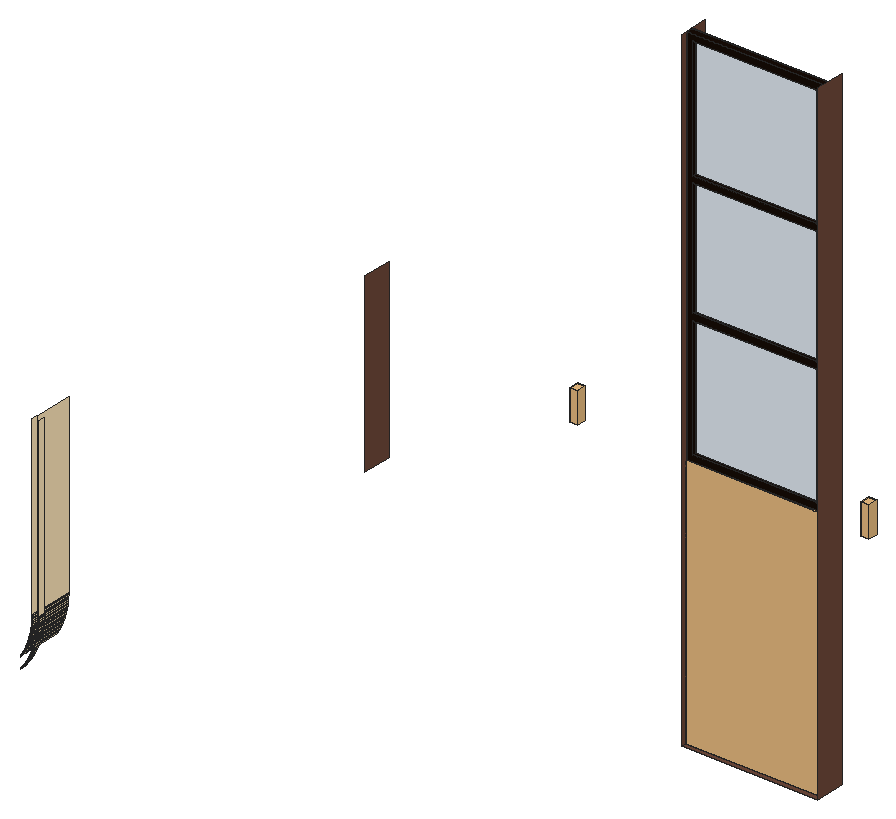
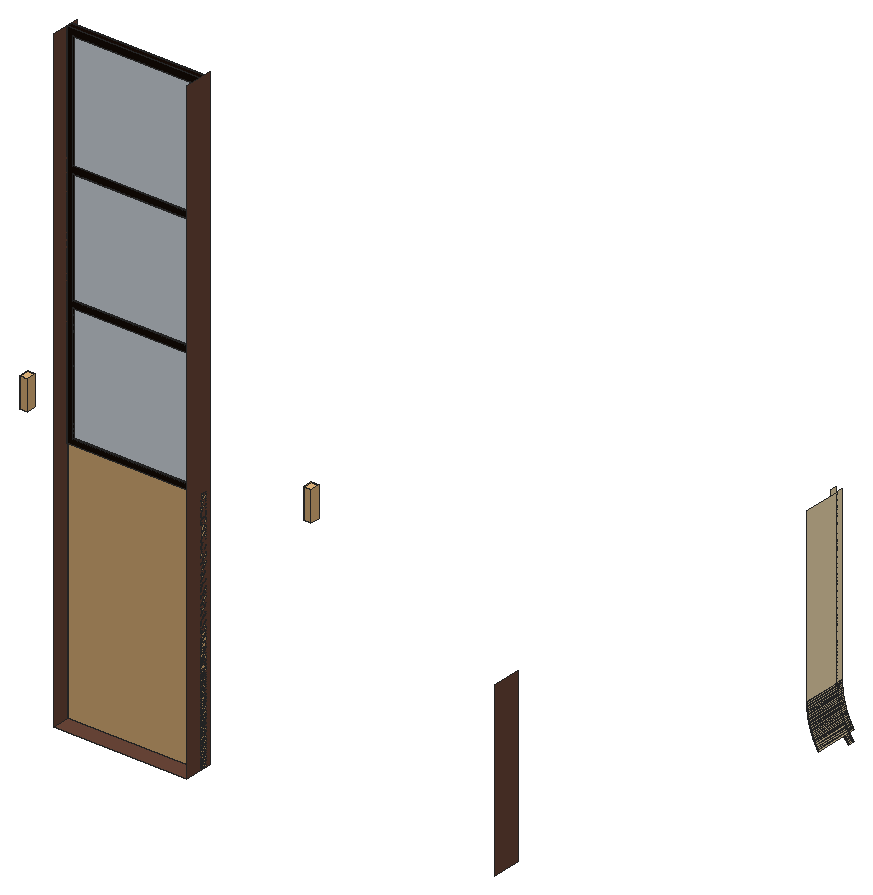
# SketchUp Ruby script. Lengths in inches.
U = 1.inch
M = Sketchup.active_model
def pt(a) = Geom::Point3d.new(a.map { |v| v * U })
def face(e, loops, mat)
  f = e.add_face(loops[0].map { |a| pt(a) })
  loops[1..].each { |l| e.add_face(l.map { |a| pt(a) }).erase! }
  f.material = f.back_material = mat if mat
  f
end
# faces: each face lists its corners as indices into pts; further lists are holes
def faces(e, pts, list, mat = nil) = list.each { |f| face(e, (f[0].is_a?(Array) ? f : [f]).map { |l| l.map { |i| pts[i] } }, mat) }
# xy, xz, yz: faces in a plane at the given z, y or x. An outline is a flat list of corners, or four numbers for a rectangle; further outlines are holes
def ring(l) = l.size == 4 ? [[l[0], l[1]], [l[2], l[1]], [l[2], l[3]], [l[0], l[3]]] : l.each_slice(2).to_a
def flat(e, list, mat, &to3) = list.each { |f| face(e, (f[0].is_a?(Array) ? f : [f]).map { |l| ring(l).map { |u, v| to3.(u, v) } }, mat) }
def xy(e, z, list, mat = nil) = flat(e, list, mat) { |x, y| [x, y, z] }
def xz(e, y, list, mat = nil) = flat(e, list, mat) { |x, z| [x, y, z] }
def yz(e, x, list, mat = nil) = flat(e, list, mat) { |y, z| [x, y, z] }
def lines(e, pts, list) = list.each { |a, b| e.add_line(pt(pts[a]), pt(pts[b])) }
# prism: a flat outline (further loops are holes) pulled along v
def prism(e, loops, v, mat = nil)
  f = face(e, loops, mat); d = Geom::Vector3d.new(v.map { |x| x * U })
  f.pushpull(f.normal.samedirection?(d) ? d.length : -d.length)
end
def box(e, o, s, mat = nil) = prism(e, [[o, [o[0] + s[0], o[1], o[2]], [o[0] + s[0], o[1] + s[1], o[2]], [o[0], o[1] + s[1], o[2]]]], [0, 0, s[2]], mat)
def at(x, y, z, deg = 0) = Geom::Transformation.translation(pt([x, y, z])) * Geom::Transformation.rotation(ORIGIN, Z_AXIS, deg.degrees)
def axes(o, x, y, z) = Geom::Transformation.new([*x, 0, *y, 0, *z, 0, *pt(o).to_a, 1])
def part(name) = M.definitions.add(name)
# library, detail: a bought-in or finely detailed component or shape, given as its bounding box
def library(name, o, s) = part(name).tap { |d| box(d.entities, o, s) }
def detail(e, o, s) = box(e.add_group.entities, o, s)
def put(e, d, t, mat = nil) = e.add_instance(d, t).tap { |i| i.material = mat if mat }
def group(e, t, mat = nil) = e.add_group.tap { |g| g.transformation = t; g.material = mat if mat }.entities
root = M.entities
M.materials.add("1026 AP 7946 SUNNY SIDE UP").color = [254, 231, 186]
M.materials.add("1916 AP K226 Macadamia Cream-N").color = [109, 72, 58]
M.materials.add("[Mirror 02]").color = [228, 237, 245]
M.materials.add("[Wood Veneer 01]").color = [23, 13, 7]
c1 = library("WALL LIGHT 69",[4.19,4.05,-9.3],[4.61,5.7,18.16])
c2 = part("1")
box(c2.entities,[0,-0.47,0],[38,0.47,35.96])
c3 = library("Glass Door",[0,0,0],[72,3.54,96])
xy(root,138,[[305.52,302,347.52,311]],"1916 AP K226 Macadamia Cream-N")
yz(root,177,[[213.1,167.53,215,167.76],[215,167.53,215.1,167.76],[215.1,167.53,227,167.76],[213.1,167.76,215,168],[215,167.76,215.1,168],
  [215.1,167.76,227,168],[213.1,168,215,222],[215,168,215.1,222],[215.1,168,227,222]],"1026 AP 7946 SUNNY SIDE UP")
yz(root,179,[[213.1,167.49,215.1,167.74],[213.1,167.74,215.1,168],[213.1,168,215.1,222]],"1026 AP 7946 SUNNY SIDE UP")
yz(root,189,[[326,162,335,216]],"1916 AP K226 Macadamia Cream-N")
yz(root,305.52,[[302,138,311,333.89]],"1916 AP K226 Macadamia Cream-N")
yz(root,347.52,[[302,138,311,333.89]],"1916 AP K226 Macadamia Cream-N")
p = [[173.42,213.1,151.9],[173.42,215.1,151.9],[173.58,215.1,152.1],[173.58,213.1,152.1],[173.73,215.1,152.31],[173.73,213.1,152.31],
  [173.88,215.1,152.51],[173.88,213.1,152.51],[174.03,215.1,152.72],[174.03,213.1,152.72],[174.18,215.1,152.92],[174.18,213.1,152.92],
  [174.33,215.1,153.13],[174.33,213.1,153.13],[174.48,215.1,153.34],[174.48,213.1,153.34],[174.62,215.1,153.56],[174.62,213.1,153.56],
  [174.76,215.1,153.77],[174.76,213.1,153.77],[174.9,215.1,153.98],[174.9,213.1,153.98],[175.03,215.1,154.2],[175.03,213.1,154.2],
  [175.17,215.1,154.42],[175.17,213.1,154.42],[175.3,215.1,154.63],[175.3,213.1,154.63],[175.43,215.1,154.85],[175.43,213.1,154.85],
  [175.56,215.1,155.07],[175.56,213.1,155.07],[175.68,215.1,155.3],[175.68,213.1,155.3],[173.46,213.1,155.46],[173.46,215,155.46],
  [173.34,215,155.26],[173.34,213.1,155.26],[175.81,215.1,155.52],[175.81,213.1,155.52],[173.34,227,155.26],[173.34,215.1,155.26],
  [173.46,215.1,155.46],[173.46,227,155.46],[173.59,213.1,155.66],[173.59,215,155.66],[175.93,215.1,155.74],[175.93,213.1,155.74],
  [173.59,215.1,155.66],[173.59,227,155.66],[173.71,213.1,155.86],[173.71,215,155.86],[176.05,215.1,155.97],[176.05,213.1,155.97],
  [173.71,215.1,155.86],[173.71,227,155.86],[173.82,213.1,156.07],[173.82,215,156.07],[173.82,215.1,156.07],[173.82,227,156.07],
  [176.17,215.1,156.2],[176.17,213.1,156.2],[173.94,213.1,156.27],[173.94,215,156.27],[173.94,215.1,156.27],[173.94,227,156.27],
  [176.28,215.1,156.42],[176.28,213.1,156.42],[174.05,213.1,156.48],[174.05,215,156.48],[174.05,215.1,156.48],[174.05,227,156.48],
  [176.39,215.1,156.65],[176.39,213.1,156.65],[174.17,213.1,156.6875],[174.17,215,156.6875],[174.17,215.1,156.6875],[174.17,227,156.6875],
  [174.28,213.1,156.89],[174.28,215,156.89],[176.5,215.1,156.88],[176.5,213.1,156.88],[174.28,215.1,156.89],[174.28,227,156.89],
  [174.38,213.1,157.1],[174.38,215,157.1],[176.61,215.1,157.11],[176.61,213.1,157.11],[174.38,215.1,157.1],[174.38,227,157.1],
  [174.49,213.1,157.31],[174.49,215,157.31],[176.72,215.1,157.35],[176.72,213.1,157.35],[174.49,215.1,157.31],[174.49,227,157.31],
  [174.59,213.1,157.53],[174.59,215,157.53],[176.82,215.1,157.58],[176.82,213.1,157.58],[174.59,215.1,157.53],[174.59,227,157.53],
  [174.7,213.1,157.74],[174.7,215,157.74],[174.7,215.1,157.74],[174.7,227,157.74],[176.92,215.1,157.81],[176.92,213.1,157.81],
  [174.8,213.1,157.95],[174.8,215,157.95],[174.8,215.1,157.95],[174.8,227,157.95],[177.02,215.1,158.05],[177.02,213.1,158.05],
  [174.89,213.1,158.17],[174.89,215,158.17],[174.89,215.1,158.17],[174.89,227,158.17],[177.12,215.1,158.29],[177.12,213.1,158.29],
  [174.99,213.1,158.38],[174.99,215,158.38],[174.99,215.1,158.38],[174.99,227,158.38],[177.21,215.1,158.52],[177.21,213.1,158.52],
  [175.08,213.1,158.6],[175.08,215,158.6],[175.08,215.1,158.6],[175.08,227,158.6],[177.3,215.1,158.76],[177.3,213.1,158.76],
  [175.17,213.1,158.82],[175.17,215,158.82],[175.17,215.1,158.82],[175.17,227,158.82],[175.26,213.1,159.03],[175.26,215,159.03],
  [177.39,215.1,159],[177.39,213.1,159],[175.26,215.1,159.03],[175.26,227,159.03],[175.35,213.1,159.25],[175.35,215,159.25],
  [177.48,215.1,159.24],[177.48,213.1,159.24],[175.35,215.1,159.25],[175.35,227,159.25],[177.56,215.1,159.48],[177.56,213.1,159.48],
  [175.43,213.1,159.47],[175.43,215,159.47],[175.43,215.1,159.47],[175.43,227,159.47],[175.52,213.1,159.69],[175.52,215,159.69],
  [177.65,215.1,159.72],[177.65,213.1,159.72],[175.52,215.1,159.69],[175.52,227,159.69],[175.6,213.1,159.91],[175.6,215,159.91],
  [177.73,215.1,159.97],[177.73,213.1,159.97],[175.6,215.1,159.91],[175.6,227,159.91],[175.68,213.1,160.14],[175.68,215,160.14],
  [175.68,215.1,160.14],[175.68,227,160.14],[177.81,215.1,160.21],[177.81,213.1,160.21],[175.75,213.1,160.36],[175.75,215,160.36],
  [175.75,215.1,160.36],[175.75,227,160.36],[177.88,215.1,160.45],[177.88,213.1,160.45],[175.83,213.1,160.58],[175.83,215,160.58],
  [175.83,215.1,160.58],[175.83,227,160.58],[177.95,215.1,160.7],[177.95,213.1,160.7],[175.9,213.1,160.81],[175.9,215,160.81],
  [175.9,215.1,160.81],[175.9,227,160.81],[178.02,215.1,160.94],[178.02,213.1,160.94],[175.97,213.1,161.03],[175.97,215,161.03],
  [175.97,215.1,161.03],[175.97,227,161.03],[178.09,215.1,161.1875],[178.09,213.1,161.1875],[176.03,213.1,161.26],[176.03,215,161.26],
  [176.03,215.1,161.26],[176.03,227,161.26],[178.16,215.1,161.44],[178.16,213.1,161.44],[176.1,213.1,161.49],[176.1,215,161.49],
  [176.1,215.1,161.49],[176.1,227,161.49],[178.22,215.1,161.68],[178.22,213.1,161.68],[176.16,213.1,161.71],[176.16,215,161.71],
  [176.16,215.1,161.71],[176.16,227,161.71],[176.22,213.1,161.94],[176.22,215,161.94],[178.28,215.1,161.93],[178.28,213.1,161.93],
  [176.22,215.1,161.94],[176.22,227,161.94],[176.28,213.1,162.17],[176.28,215,162.17],[178.34,215.1,162.18],[178.34,213.1,162.18],
  [176.28,215.1,162.17],[176.28,227,162.17],[176.34,213.1,162.4],[176.34,215,162.4],[178.4,215.1,162.43],[178.4,213.1,162.43],
  [176.34,215.1,162.4],[176.34,227,162.4],[176.39,213.1,162.625],[176.39,215,162.625],[178.45,215.1,162.68],[178.45,213.1,162.68],
  [176.39,215.1,162.625],[176.39,227,162.625],[176.44,213.1,162.86],[176.44,215,162.86],[176.44,215.1,162.86],[176.44,227,162.86],
  [178.5,215.1,162.93],[178.5,213.1,162.93],[176.49,213.1,163.09],[176.49,215,163.09],[178.55,215.1,163.18],[178.55,213.1,163.18],
  [176.49,215.1,163.09],[176.49,227,163.09],[176.54,213.1,163.32],[176.54,215,163.32],[176.54,215.1,163.32],[176.54,227,163.32],
  [178.6,215.1,163.43],[178.6,213.1,163.43],[176.58,213.1,163.55],[176.58,215,163.55],[176.58,215.1,163.55],[176.58,227,163.55],
  [178.64,215.1,163.68],[178.64,213.1,163.68],[176.625,213.1,163.78],[176.625,215,163.78],[176.625,215.1,163.78],[176.625,227,163.78],
  [178.68,215.1,163.93],[178.68,213.1,163.93],[176.67,213.1,164.01],[176.67,215,164.01],[176.67,215.1,164.01],[176.67,227,164.01],
  [178.72,215.1,164.19],[178.72,213.1,164.19],[176.7,213.1,164.25],[176.7,215,164.25],[176.7,215.1,164.25],[176.7,227,164.25],
  [176.74,213.1,164.48],[176.74,215,164.48],[178.75,215.1,164.4375],[178.75,213.1,164.4375],[176.74,215.1,164.48],[176.74,227,164.48],
  [178.79,215.1,164.69],[178.79,213.1,164.69],[176.77,213.1,164.71],[176.77,215,164.71],[176.77,215.1,164.71],[176.77,227,164.71],
  [176.8,213.1,164.95],[176.8,215,164.95],[178.82,215.1,164.94],[178.82,213.1,164.94],[176.8,215.1,164.95],[176.8,227,164.95],
  [176.83,213.1,165.18],[176.83,215,165.18],[178.85,215.1,165.2],[178.85,213.1,165.2],[176.83,215.1,165.18],[176.83,227,165.18],
  [176.86,213.1,165.41],[176.86,215,165.41],[178.875,215.1,165.45],[178.875,213.1,165.45],[176.86,215.1,165.41],[176.86,227,165.41],
  [176.88,213.1,165.65],[176.88,215,165.65],[176.88,215.1,165.65],[176.88,227,165.65],[178.9,215.1,165.71],[178.9,213.1,165.71],
  [176.91,213.1,165.88],[176.91,215,165.88],[176.91,215.1,165.88],[176.91,227,165.88],[178.92,215.1,165.96],[178.92,213.1,165.96],
  [176.93,213.1,166.12],[176.93,215,166.12],[176.93,215.1,166.12],[176.93,227,166.12],[178.9375,215.1,166.21],[178.9375,213.1,166.21],
  [176.94,213.1,166.35],[176.94,215,166.35],[176.94,215.1,166.35],[176.94,227,166.35],[178.95,215.1,166.47],[178.95,213.1,166.47],
  [176.96,213.1,166.59],[176.96,215,166.59],[176.96,215.1,166.59],[176.96,227,166.59],[178.97,215.1,166.72],[178.97,213.1,166.72],
  [176.97,213.1,166.82],[176.97,215,166.82],[176.97,215.1,166.82],[176.97,227,166.82],[178.98,215.1,166.98],[178.98,213.1,166.98],
  [176.98,213.1,167.06],[176.98,215,167.06],[176.98,215.1,167.06],[176.98,227,167.06],[178.99,215.1,167.23],[178.99,213.1,167.23],
  [176.99,213.1,167.29],[176.99,215,167.29],[176.99,215.1,167.29],[176.99,227,167.29],[179,215.1,167.49],[179,213.1,167.49],
  [177,213.1,167.53],[177,215,167.53],[177,215.1,167.53],[177,227,167.53]]
faces(root,p,[[0,1,2,3],[3,2,4,5],[5,4,6,7],[7,6,8,9],[9,8,10,11],[11,10,12,13],[13,12,14,15],[15,14,16,17],
  [17,16,18,19],[19,18,20,21],[21,20,22,23],[23,22,24,25],[25,24,26,27],[27,26,28,29],[29,28,30,31],[31,30,32,33],
  [34,35,36,37],[33,32,38,39],[40,41,42,43],[44,45,35,34],[39,38,46,47],[42,35,45,48],[43,42,48,49],[50,51,45,44],
  [47,46,52,53],[48,45,51,54],[49,48,54,55],[56,57,51,50],[54,51,57,58],[55,54,58,59],[53,52,60,61],[62,63,57,56],
  [58,57,63,64],[59,58,64,65],[61,60,66,67],[68,69,63,62],[64,63,69,70],[65,64,70,71],[67,66,72,73],[74,75,69,68],
  [70,69,75,76],[71,70,76,77],[78,79,75,74],[73,72,80,81],[76,75,79,82],[77,76,82,83],[84,85,79,78],[81,80,86,87],
  [82,79,85,88],[83,82,88,89],[90,91,85,84],[87,86,92,93],[88,85,91,94],[89,88,94,95],[96,97,91,90],[93,92,98,99],
  [94,91,97,100],[95,94,100,101],[102,103,97,96],[100,97,103,104],[101,100,104,105],[99,98,106,107],[108,109,103,102],[104,103,109,110],
  [105,104,110,111],[107,106,112,113],[114,115,109,108],[110,109,115,116],[111,110,116,117],[113,112,118,119],[120,121,115,114],[116,115,121,122],
  [117,116,122,123],[119,118,124,125],[126,127,121,120],[122,121,127,128],[123,122,128,129],[125,124,130,131],[132,133,127,126],[128,127,133,134],
  [129,128,134,135],[136,137,133,132],[131,130,138,139],[134,133,137,140],[135,134,140,141],[142,143,137,136],[139,138,144,145],[140,137,143,146],
  [141,140,146,147],[145,144,148,149],[150,151,143,142],[146,143,151,152],[147,146,152,153],[154,155,151,150],[149,148,156,157],[152,151,155,158],
  [153,152,158,159],[160,161,155,154],[157,156,162,163],[158,155,161,164],[159,158,164,165],[166,167,161,160],[164,161,167,168],[165,164,168,169],
  [163,162,170,171],[172,173,167,166],[168,167,173,174],[169,168,174,175],[171,170,176,177],[178,179,173,172],[174,173,179,180],[175,174,180,181],
  [177,176,182,183],[184,185,179,178],[180,179,185,186],[181,180,186,187],[183,182,188,189],[190,191,185,184],[186,185,191,192],[187,186,192,193],
  [189,188,194,195],[196,197,191,190],[192,191,197,198],[193,192,198,199],[195,194,200,201],[202,203,197,196],[198,197,203,204],[199,198,204,205],
  [201,200,206,207],[208,209,203,202],[204,203,209,210],[205,204,210,211],[212,213,209,208],[207,206,214,215],[210,209,213,216],[211,210,216,217],
  [218,219,213,212],[215,214,220,221],[216,213,219,222],[217,216,222,223],[224,225,219,218],[221,220,226,227],[222,219,225,228],[223,222,228,229],
  [230,231,225,224],[227,226,232,233],[228,225,231,234],[229,228,234,235],[236,237,231,230],[234,231,237,238],[235,234,238,239],[233,232,240,241],
  [242,243,237,236],[241,240,244,245],[238,237,243,246],[239,238,246,247],[248,249,243,242],[246,243,249,250],[247,246,250,251],[245,244,252,253],
  [254,255,249,248],[250,249,255,256],[251,250,256,257],[253,252,258,259],[260,261,255,254],[256,255,261,262],[257,256,262,263],[259,258,264,265],
  [266,267,261,260],[262,261,267,268],[263,262,268,269],[265,264,270,271],[272,273,267,266],[268,267,273,274],[269,268,274,275],[276,277,273,272],
  [271,270,278,279],[274,273,277,280],[275,274,280,281],[279,278,282,283],[284,285,277,276],[280,277,285,286],[281,280,286,287],[288,289,285,284],
  [283,282,290,291],[286,285,289,292],[287,286,292,293],[294,295,289,288],[291,290,296,297],[292,289,295,298],[293,292,298,299],[300,301,295,294],
  [297,296,302,303],[298,295,301,304],[299,298,304,305],[306,307,301,300],[304,301,307,308],[305,304,308,309],[303,302,310,311],[312,313,307,306],
  [308,307,313,314],[309,308,314,315],[311,310,316,317],[318,319,313,312],[314,313,319,320],[315,314,320,321],[317,316,322,323],[324,325,319,318],
  [320,319,325,326],[321,320,326,327],[323,322,328,329],[330,331,325,324],[326,325,331,332],[327,326,332,333],[329,328,334,335],[336,337,331,330],
  [332,331,337,338],[333,332,338,339],[335,334,340,341],[342,343,337,336],[338,337,343,344],[339,338,344,345],[341,340,346,347],[348,349,343,342],
  [344,343,349,350],[345,344,350,351],[347,346,352,353],[354,355,349,348],[350,349,355,356],[351,350,356,357]],"1026 AP 7946 SUNNY SIDE UP")
put(root,c1,axes([271.51,296.68,222.25],[0.52,0,0],[0,0.52,0],[0,0,0.52]))
g1 = group(root,at(305.52,302,138),"[Wood Veneer 01]")
g2 = group(g1,at(0,4,78))
prism(g2,[[[42,-2,117.89],[0,-2,117.89],[0,-2,0],[42,-2,0]],[[40,-2,115.89],[40,-2,78.93],[2,-2,78.93],[2,-2,115.89]],[[2,-2,38.96],[40,-2,38.96],[40,-2,2],[2,-2,2]],[[40,-2,76.93],[40,-2,40.96],[2,-2,40.96],[2,-2,76.93]]],[0,2,0])
put(g2,c2,at(2,-0.53,40.96),"[Mirror 02]")
put(g2,c2,axes([2,-0.53,2],[1,0,0],[0,1,0],[0,0,1.02781]),"[Mirror 02]")
put(g2,c2,axes([2,-0.53,78.93],[1,0,0],[0,1,0],[0,0,1.02781]),"[Mirror 02]")
put(root,c3,axes([305.52,303.52,138],[0.58333,0,0],[0,0.57,0],[0,0,0.8125]))
put(root,c1,axes([361.01,296.68,222.25],[0.52,0,0],[0,0.52,0],[0,0,0.52]))
